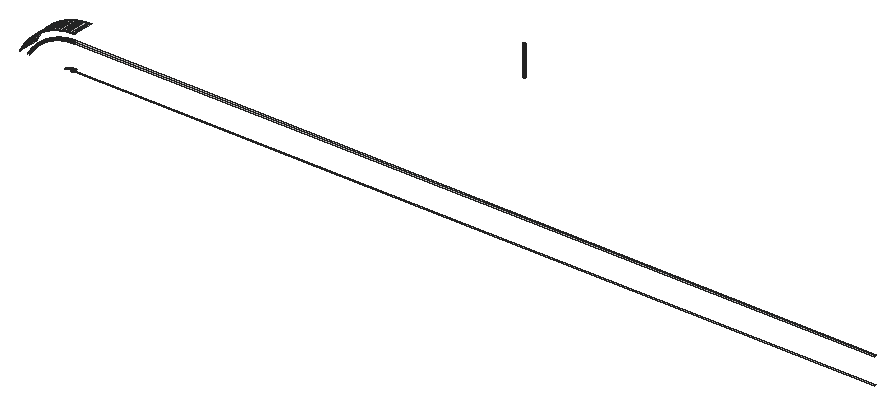
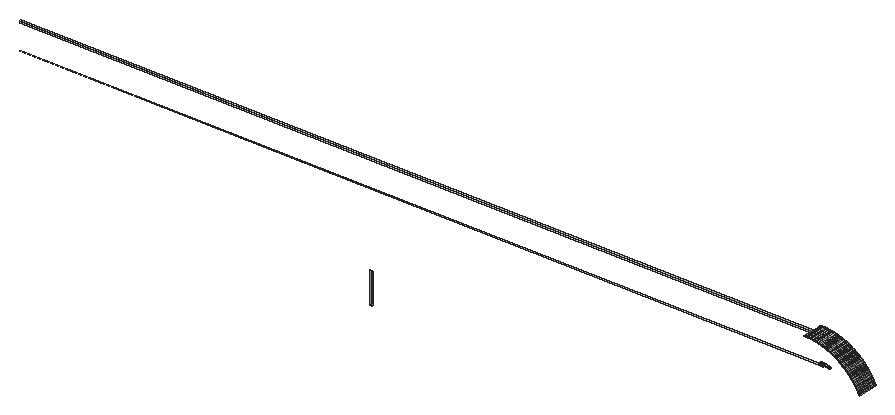
# SketchUp Ruby script. Lengths in inches.
U = 1.inch
M = Sketchup.active_model
def pt(a) = Geom::Point3d.new(a.map { |v| v * U })
def face(e, loops, mat)
  f = e.add_face(loops[0].map { |a| pt(a) })
  loops[1..].each { |l| e.add_face(l.map { |a| pt(a) }).erase! }
  f.material = f.back_material = mat if mat
  f
end
# faces: each face lists its corners as indices into pts; further lists are holes
def faces(e, pts, list, mat = nil) = list.each { |f| face(e, (f[0].is_a?(Array) ? f : [f]).map { |l| l.map { |i| pts[i] } }, mat) }
# xy, xz, yz: faces in a plane at the given z, y or x. An outline is a flat list of corners, or four numbers for a rectangle; further outlines are holes
def ring(l) = l.size == 4 ? [[l[0], l[1]], [l[2], l[1]], [l[2], l[3]], [l[0], l[3]]] : l.each_slice(2).to_a
def flat(e, list, mat, &to3) = list.each { |f| face(e, (f[0].is_a?(Array) ? f : [f]).map { |l| ring(l).map { |u, v| to3.(u, v) } }, mat) }
def xy(e, z, list, mat = nil) = flat(e, list, mat) { |x, y| [x, y, z] }
def xz(e, y, list, mat = nil) = flat(e, list, mat) { |x, z| [x, y, z] }
def yz(e, x, list, mat = nil) = flat(e, list, mat) { |y, z| [x, y, z] }
def lines(e, pts, list) = list.each { |a, b| e.add_line(pt(pts[a]), pt(pts[b])) }
# prism: a flat outline (further loops are holes) pulled along v
def prism(e, loops, v, mat = nil)
  f = face(e, loops, mat); d = Geom::Vector3d.new(v.map { |x| x * U })
  f.pushpull(f.normal.samedirection?(d) ? d.length : -d.length)
end
def box(e, o, s, mat = nil) = prism(e, [[o, [o[0] + s[0], o[1], o[2]], [o[0] + s[0], o[1] + s[1], o[2]], [o[0], o[1] + s[1], o[2]]]], [0, 0, s[2]], mat)
def at(x, y, z, deg = 0) = Geom::Transformation.translation(pt([x, y, z])) * Geom::Transformation.rotation(ORIGIN, Z_AXIS, deg.degrees)
def axes(o, x, y, z) = Geom::Transformation.new([*x, 0, *y, 0, *z, 0, *pt(o).to_a, 1])
def part(name) = M.definitions.add(name)
# library, detail: a bought-in or finely detailed component or shape, given as its bounding box
def library(name, o, s) = part(name).tap { |d| box(d.entities, o, s) }
def detail(e, o, s) = box(e.add_group.entities, o, s)
def put(e, d, t, mat = nil) = e.add_instance(d, t).tap { |i| i.material = mat if mat }
def group(e, t, mat = nil) = e.add_group.tap { |g| g.transformation = t; g.material = mat if mat }.entities
root = M.entities
M.materials.add("[Quartz Light Brown]").color = [215, 212, 212]
xy(root,99.98,[[35.12,38,35.25,39]],"[Quartz Light Brown]")
xy(root,99.99,[[35.37,38,35.5,39]],"[Quartz Light Brown]")
xy(root,100,[[35.625,38,35.75,39],[35.75,38,35.875,39],[35.875,38,36.04,39],[36.04,38,503.96,39]],"[Quartz Light Brown]")
xy(root,100.97,[[34.93,38,35.07,39]],"[Quartz Light Brown]")
xy(root,100.99,[[35.33,38,35.47,39]],"[Quartz Light Brown]")
xy(root,101,[[35.6,38,35.73,39],[35.73,38,35.87,39],[35.87,38,36.04,39]],"[Quartz Light Brown]")
xy(root,114.98,[[34.78,38,35.03,39]],"[Quartz Light Brown]")
xy(root,115,[[35.51,38,35.76,39],[35.76,38,36.01,39],[36.01,38,503.99,39]],"[Quartz Light Brown]")
xy(root,115.98,[[34.74,38,34.99,39]],"[Quartz Light Brown]")
xy(root,116,[[35.5,38,35.75,39],[35.75,38,36.01,39],[36.01,38,503.99,39]],"[Quartz Light Brown]")
xy(root,120,[[35.43,38,35.72,50],[35.72,38,36,50]],"[Quartz Light Brown]")
xz(root,143,[[215.8,114,216,132]],"[Quartz Light Brown]")
xz(root,143.01,[[215.41,114,215.61,132]],"[Quartz Light Brown]")
p = [[3.67,38,99.84],[3.8,38,100.09],[3.8,50,100.09],[3.67,50,99.84],[9.32,39,99.78],[9.32,38,99.78],
  [9.44,38,99.99],[9.44,39,99.99],[29.74,38,99.81],[29.74,39,99.81],[29.87,39,99.85],[29.87,38,99.85],
  [33.25,39,99.76],[33.25,38,99.76],[33.375,38,99.78],[33.375,39,99.78],[33.5,38,99.8],[33.5,39,99.8],
  [33.62,38,99.82],[33.62,39,99.82],[33.75,38,99.84],[33.75,39,99.84],[33.87,38,99.86],[33.87,39,99.86],
  [8.2,38,99.85],[8.2,39,99.85],[8.33,39,100.07],[8.33,38,100.07],[29.99,39,99.9],[29.99,38,99.9],
  [30.12,39,99.95],[30.12,38,99.95],[30.24,39,99.99],[30.24,38,99.99],[33.99,38,99.875],[33.99,39,99.875],
  [34.12,38,99.89],[34.12,39,99.89],[34.24,38,99.9],[34.24,39,99.9],[34.37,38,99.92],[34.37,39,99.92],
  [34.49,38,99.93],[34.49,39,99.93],[34.62,38,99.94],[34.62,39,99.94],[34.74,38,99.95],[34.74,39,99.95],
  [9.57,38,100.2],[9.57,39,100.2],[30.37,39,100.04],[30.37,38,100.04],[30.49,39,100.08],[30.49,38,100.08],
  [34.87,38,99.96],[34.87,39,99.96],[35,38,99.97],[35,39,99.97],[35.12,38,99.98],[35.12,39,99.98],
  [35.25,39,99.98],[35.25,38,99.98],[35.37,38,99.99],[35.37,39,99.99],[35.5,39,99.99],[35.5,38,99.99],
  [35.625,38,100],[35.625,39,100],[3.92,38,100.34],[3.92,50,100.34],[8.46,39,100.29],[8.46,38,100.29],
  [30.62,39,100.125],[30.62,38,100.125],[30.75,39,100.17],[30.75,38,100.17],[9.7,38,100.4],[9.7,39,100.4],
  [30.875,39,100.21],[30.875,38,100.21],[31,39,100.25],[31,38,100.25],[31.13,39,100.29],[31.13,38,100.29],
  [4.05,38,100.6],[4.05,50,100.6],[8.59,39,100.51],[8.59,38,100.51],[31.26,39,100.32],[31.26,38,100.32],
  [31.39,39,100.36],[31.39,38,100.36],[9.83,38,100.61],[9.83,39,100.61],[31.51,39,100.4],[31.51,38,100.4],
  [31.64,39,100.43],[31.64,38,100.43],[31.77,39,100.47],[31.77,38,100.47],[8.72,39,100.72],[8.72,38,100.72],
  [31.9,39,100.5],[31.9,38,100.5],[32.03,39,100.53],[32.03,38,100.53],[32.16,39,100.5625],[32.16,38,100.5625],
  [4.18,38,100.85],[4.18,50,100.85],[9.96,38,100.82],[9.96,39,100.82],[32.29,39,100.59],[32.29,38,100.59],
  [32.42,39,100.62],[32.42,38,100.62],[32.55,39,100.65],[32.55,38,100.65],[32.68,39,100.67],[32.68,38,100.67],
  [8.85,39,100.93],[8.85,38,100.93],[32.81,39,100.7],[32.81,38,100.7],[32.95,39,100.72],[32.95,38,100.72],
  [33.08,39,100.75],[33.08,38,100.75],[33.21,39,100.77],[33.21,38,100.77],[4.32,38,101.09],[4.32,50,101.09],
  [10.09,38,101.02],[10.09,39,101.02],[33.34,39,100.79],[33.34,38,100.79],[33.47,39,100.8125],[33.47,38,100.8125],
  [33.6,39,100.83],[33.6,38,100.83],[33.74,39,100.85],[33.74,38,100.85],[33.87,39,100.87],[33.87,38,100.87],
  [8.98,39,101.15],[8.98,38,101.15],[34,39,100.88],[34,38,100.88],[34.13,39,100.9],[34.13,38,100.9],
  [34.27,39,100.91],[34.27,38,100.91],[34.4,39,100.92],[34.4,38,100.92],[34.53,39,100.9375],[34.53,38,100.9375],
  [34.67,39,100.95],[34.67,38,100.95],[34.8,39,100.96],[34.8,38,100.96],[10.22,38,101.22],[10.22,39,101.22],
  [34.93,39,100.97],[34.93,38,100.97],[35.07,38,100.97],[35.07,39,100.97],[35.2,39,100.98],[35.2,38,100.98],
  [35.33,39,100.99],[35.33,38,100.99],[35.47,38,100.99],[35.47,39,100.99],[35.6,39,101],[35.6,38,101],
  [4.45,38,101.34],[4.45,50,101.34],[9.12,39,101.36],[9.12,38,101.36],[10.36,38,101.42],[10.36,39,101.42],
  [4.59,38,101.59],[4.59,50,101.59],[9.25,39,101.57],[9.25,38,101.57],[10.5,38,101.625],[10.5,39,101.625],
  [4.73,38,101.84],[4.73,50,101.84],[9.39,39,101.78],[9.39,38,101.78],[10.64,38,101.83],[10.64,39,101.83],
  [4.87,38,102.08],[4.87,50,102.08],[9.53,39,101.99],[9.53,38,101.99],[10.78,38,102.02],[10.78,39,102.02],
  [9.68,39,102.19],[9.68,38,102.19],[10.92,38,102.22],[10.92,39,102.22],[5.01,38,102.33],[5.01,50,102.33],
  [9.82,39,102.4],[9.82,38,102.4],[11.0625,38,102.42],[11.0625,39,102.42],[5.16,38,102.57],[5.16,50,102.57],
  [9.96,39,102.61],[9.96,38,102.61],[11.21,38,102.61],[11.21,39,102.61],[5.3,38,102.81],[5.3,50,102.81],
  [10.11,39,102.81],[10.11,38,102.81],[11.36,38,102.81],[11.36,39,102.81],[5.45,38,103.05],[5.45,50,103.05],
  [10.26,39,103.01],[10.26,38,103.01],[11.51,38,103],[11.51,39,103],[10.41,39,103.21],[10.41,38,103.21],
  [11.66,38,103.19],[11.66,39,103.19],[5.6,38,103.29],[5.6,50,103.29],[10.5625,39,103.41],[10.5625,38,103.41],
  [11.81,38,103.38],[11.81,39,103.38],[5.76,38,103.53],[5.76,50,103.53],[10.72,39,103.61],[10.72,38,103.61],
  [11.96,38,103.57],[11.96,39,103.57],[5.91,38,103.76],[5.91,50,103.76],[10.87,39,103.8125],[10.87,38,103.8125],
  [12.11,38,103.76],[12.11,39,103.76],[6.07,38,104],[6.07,50,104],[11.03,39,104.01],[11.03,38,104.01],
  [12.27,38,103.95],[12.27,39,103.95],[12.43,38,104.13],[12.43,39,104.13],[6.23,38,104.24],[6.23,50,104.24],
  [11.18,39,104.2],[11.18,38,104.2],[12.59,38,104.32],[12.59,39,104.32],[6.38,38,104.47],[6.38,50,104.47],
  [11.34,39,104.4],[11.34,38,104.4],[12.75,38,104.5],[12.75,39,104.5],[11.5,39,104.59],[11.5,38,104.59],
  [6.55,38,104.7],[6.55,50,104.7],[12.91,38,104.68],[12.91,39,104.68],[11.67,39,104.78],[11.67,38,104.78],
  [6.71,38,104.93],[6.71,50,104.93],[13.07,38,104.86],[13.07,39,104.86],[11.83,39,104.97],[11.83,38,104.97],
  [6.875,38,105.16],[6.875,50,105.16],[13.24,38,105.04],[13.24,39,105.04],[12,39,105.16],[12,38,105.16],
  [13.4,38,105.22],[13.4,39,105.22],[7.04,38,105.39],[7.04,50,105.39],[12.16,39,105.35],[12.16,38,105.35],
  [13.57,38,105.4],[13.57,39,105.4],[12.33,39,105.54],[12.33,38,105.54],[7.21,38,105.62],[7.21,50,105.62],
  [13.74,38,105.57],[13.74,39,105.57],[12.5,39,105.72],[12.5,38,105.72],[7.38,38,105.84],[7.38,50,105.84],
  [13.91,38,105.75],[13.91,39,105.75],[12.67,39,105.91],[12.67,38,105.91],[14.08,38,105.92],[14.08,39,105.92],
  [7.55,38,106.06],[7.55,50,106.06],[12.85,39,106.09],[12.85,38,106.09],[14.25,38,106.09],[14.25,39,106.09],
  [7.73,38,106.29],[7.73,50,106.29],[13.02,39,106.27],[13.02,38,106.27],[14.43,38,106.26],[14.43,39,106.26],
  [7.9,38,106.51],[7.9,50,106.51],[13.2,39,106.45],[13.2,38,106.45],[14.6,38,106.43],[14.6,39,106.43],
  [13.37,39,106.63],[13.37,38,106.63],[14.78,38,106.6],[14.78,39,106.6],[8.08,38,106.73],[8.08,50,106.73],
  [13.55,39,106.8],[13.55,38,106.8],[14.96,38,106.76],[14.96,39,106.76],[8.26,38,106.95],[8.26,50,106.95],
  [13.73,39,106.98],[13.73,38,106.98],[15.14,38,106.93],[15.14,39,106.93],[8.44,38,107.16],[8.44,50,107.16],
  [15.32,38,107.09],[15.32,39,107.09],[13.91,39,107.15],[13.91,38,107.15],[15.5,38,107.25],[15.5,39,107.25],
  [8.625,38,107.38],[8.625,50,107.38],[14.09,39,107.33],[14.09,38,107.33],[14.28,39,107.5],[14.28,38,107.5],
  [15.68,38,107.41],[15.68,39,107.41],[8.81,38,107.59],[8.81,50,107.59],[15.87,38,107.57],[15.87,39,107.57],
  [14.46,39,107.67],[14.46,38,107.67],[9,38,107.81],[9,50,107.81],[16.05,38,107.73],[16.05,39,107.73],
  [14.65,39,107.84],[14.65,38,107.84],[16.24,38,107.89],[16.24,39,107.89],[9.18,38,108.02],[9.18,50,108.02],
  [14.84,39,108],[14.84,38,108],[16.43,38,108.04],[16.43,39,108.04],[9.375,38,108.23],[9.375,50,108.23],
  [15.03,39,108.17],[15.03,38,108.17],[16.62,38,108.19],[16.62,39,108.19],[9.5625,38,108.4375],[9.5625,50,108.4375],
  [15.22,39,108.33],[15.22,38,108.33],[16.81,38,108.34],[16.81,39,108.34],[15.41,39,108.5],[15.41,38,108.5],
  [17,38,108.49],[17,39,108.49],[9.76,38,108.64],[9.76,50,108.64],[15.6,39,108.66],[15.6,38,108.66],
  [17.19,38,108.64],[17.19,39,108.64],[9.95,38,108.85],[9.95,50,108.85],[17.39,38,108.79],[17.39,39,108.79],
  [15.8,39,108.82],[15.8,38,108.82],[10.15,38,109.05],[10.15,50,109.05],[15.99,39,108.97],[15.99,38,108.97],
  [17.58,38,108.9375],[17.58,39,108.9375],[17.78,38,109.08],[17.78,39,109.08],[16.1875,39,109.13],[16.1875,38,109.13],
  [10.35,38,109.26],[10.35,50,109.26],[16.39,39,109.28],[16.39,38,109.28],[17.98,38,109.22],[17.98,39,109.22],
  [18.17,38,109.36],[18.17,39,109.36],[10.54,38,109.46],[10.54,50,109.46],[16.59,39,109.4375],[16.59,38,109.4375],
  [16.79,39,109.59],[16.79,38,109.59],[18.375,38,109.5],[18.375,39,109.5],[10.74,38,109.65],[10.74,50,109.65],
  [18.58,38,109.64],[18.58,39,109.64],[16.99,39,109.74],[16.99,38,109.74],[18.78,38,109.78],[18.78,39,109.78],
  [10.95,38,109.85],[10.95,50,109.85],[17.19,39,109.89],[17.19,38,109.89],[18.98,38,109.91],[18.98,39,109.91],
  [11.15,38,110.05],[11.15,50,110.05],[17.39,39,110.04],[17.39,38,110.04],[19.18,38,110.04],[19.18,39,110.04],
  [11.36,38,110.24],[11.36,50,110.24],[17.6,39,110.18],[17.6,38,110.18],[19.39,38,110.17],[19.39,39,110.17],
  [11.5625,38,110.4375],[11.5625,50,110.4375],[17.81,39,110.32],[17.81,38,110.32],[19.6,38,110.3],[19.6,39,110.3],
  [18.01,39,110.47],[18.01,38,110.47],[19.8,38,110.43],[19.8,39,110.43],[11.77,38,110.625],[11.77,50,110.625],
  [20.01,38,110.56],[20.01,39,110.56],[18.22,39,110.61],[18.22,38,110.61],[11.98,38,110.82],[11.98,50,110.82],
  [18.43,39,110.75],[18.43,38,110.75],[20.22,38,110.68],[20.22,39,110.68],[18.64,39,110.88],[18.64,38,110.88],
  [20.43,38,110.81],[20.43,39,110.81],[12.19,38,111],[12.19,50,111],[20.64,38,110.93],[20.64,39,110.93],
  [18.85,39,111.02],[18.85,38,111.02],[20.85,38,111.05],[20.85,39,111.05],[12.41,38,111.19],[12.41,50,111.19],
  [19.07,39,111.15],[19.07,38,111.15],[21.07,38,111.17],[21.07,39,111.17],[12.62,38,111.375],[12.62,50,111.375],
  [19.28,39,111.28],[19.28,38,111.28],[21.28,38,111.28],[21.28,39,111.28],[19.49,39,111.41],[19.49,38,111.41],
  [21.49,38,111.4],[21.49,39,111.4],[12.84,38,111.56],[12.84,50,111.56],[19.71,39,111.54],[19.71,38,111.54],
  [21.71,38,111.51],[21.71,39,111.51],[19.93,39,111.67],[19.93,38,111.67],[21.93,38,111.62],[21.93,39,111.62],
  [13.05,38,111.74],[13.05,50,111.74],[22.14,38,111.73],[22.14,39,111.73],[13.27,38,111.92],[13.27,50,111.92],
  [20.15,39,111.8],[20.15,38,111.8],[22.36,38,111.84],[22.36,39,111.84],[20.36,39,111.92],[20.36,38,111.92],
  [22.58,38,111.95],[22.58,39,111.95],[13.49,38,112.1],[13.49,50,112.1],[20.58,39,112.04],[20.58,38,112.04],
  [22.8,38,112.05],[22.8,39,112.05],[20.8,39,112.16],[20.8,38,112.16],[23.02,38,112.15],[23.02,39,112.15],
  [13.71,38,112.27],[13.71,50,112.27],[21.03,39,112.28],[21.03,38,112.28],[23.24,38,112.25],[23.24,39,112.25],
  [13.94,38,112.45],[13.94,50,112.45],[21.25,39,112.4],[21.25,38,112.4],[23.47,38,112.35],[23.47,39,112.35],
  [14.16,38,112.62],[14.16,50,112.62],[21.47,39,112.51],[21.47,38,112.51],[23.6875,38,112.45],[23.6875,39,112.45],
  [21.7,39,112.625],[21.7,38,112.625],[23.91,38,112.55],[23.91,39,112.55],[24.14,38,112.64],[24.14,39,112.64],
  [14.38,38,112.79],[14.38,50,112.79],[21.92,39,112.74],[21.92,38,112.74],[24.36,38,112.73],[24.36,39,112.73],
  [22.15,39,112.85],[22.15,38,112.85],[24.59,38,112.82],[24.59,39,112.82],[14.61,38,112.96],[14.61,50,112.96],
  [22.375,39,112.95],[22.375,38,112.95],[24.81,38,112.91],[24.81,39,112.91],[25.04,38,113],[25.04,39,113],
  [14.84,38,113.125],[14.84,50,113.125],[22.6,39,113.0625],[22.6,38,113.0625],[25.27,38,113.08],[25.27,39,113.08],
  [15.07,38,113.29],[15.07,50,113.29],[22.83,39,113.16],[22.83,38,113.16],[25.5,38,113.17],[25.5,39,113.17],
  [23.0625,39,113.27],[23.0625,38,113.27],[25.73,38,113.25],[25.73,39,113.25],[25.96,38,113.33],[25.96,39,113.33],
  [15.3,38,113.45],[15.3,50,113.45],[23.29,39,113.37],[23.29,38,113.37],[26.1875,38,113.41],[26.1875,39,113.41],
  [23.52,39,113.47],[23.52,38,113.47],[26.42,38,113.48],[26.42,39,113.48],[15.53,38,113.62],[15.53,50,113.62],
  [23.75,39,113.5625],[23.75,38,113.5625],[26.65,38,113.56],[26.65,39,113.56],[15.76,38,113.77],[15.76,50,113.77],
  [23.99,39,113.66],[23.99,38,113.66],[26.88,38,113.63],[26.88,39,113.63],[27.12,38,113.7],[27.12,39,113.7],
  [24.22,39,113.75],[24.22,38,113.75],[27.35,38,113.77],[27.35,39,113.77],[16,38,113.93],[16,50,113.93],
  [24.45,39,113.84],[24.45,38,113.84],[24.6875,39,113.93],[24.6875,38,113.93],[27.59,38,113.84],[27.59,39,113.84],
  [27.82,38,113.9],[27.82,39,113.9],[16.24,38,114.09],[16.24,50,114.09],[24.92,39,114.02],[24.92,38,114.02],
  [28.06,38,113.96],[28.06,39,113.96],[25.16,39,114.11],[25.16,38,114.11],[28.29,38,114.03],[28.29,39,114.03],
  [28.53,38,114.09],[28.53,39,114.09],[214.63,143.0625,132],[214.63,143.0625,114],[214.82,143.05,114],[214.82,143.05,132],
  [215.02,143.03,114],[215.02,143.03,132],[215.21,143.02,114],[215.21,143.02,132],[215.41,143.01,114],[215.41,143.01,132],
  [215.61,143.01,132],[215.61,143.01,114],[215.8,143,114],[215.8,143,132],[213.85,143.16,132],[213.85,143.16,114],
  [214.04,143.13,114],[214.04,143.13,132],[214.24,143.1,114],[214.24,143.1,132],[214.43,143.08,114],[214.43,143.08,132],
  [16.47,38,114.24],[16.47,50,114.24],[25.4,39,114.19],[25.4,38,114.19],[28.76,38,114.14],[28.76,39,114.14],
  [29,38,114.2],[29,39,114.2],[16.71,38,114.4],[16.71,50,114.4],[25.63,39,114.27],[25.63,38,114.27],
  [29.24,38,114.25],[29.24,39,114.25],[25.87,39,114.36],[25.87,38,114.36],[29.48,38,114.31],[29.48,39,114.31],
  [29.71,38,114.36],[29.71,39,114.36],[16.95,38,114.55],[16.95,50,114.55],[26.11,39,114.43],[26.11,38,114.43],
  [26.35,39,114.51],[26.35,38,114.51],[29.95,38,114.4],[29.95,39,114.4],[30.19,38,114.45],[30.19,39,114.45],
  [17.19,38,114.7],[17.19,50,114.7],[26.59,39,114.59],[26.59,38,114.59],[30.43,38,114.5],[30.43,39,114.5],
  [30.67,38,114.54],[30.67,39,114.54],[30.91,38,114.58],[30.91,39,114.58],[26.83,39,114.66],[26.83,38,114.66],
  [31.15,38,114.62],[31.15,39,114.62],[31.39,38,114.66],[31.39,39,114.66],[17.43,38,114.84],[17.43,50,114.84],
  [27.07,39,114.73],[27.07,38,114.73],[27.3125,39,114.8],[27.3125,38,114.8],[31.63,38,114.69],[31.63,39,114.69],
  [31.875,38,114.72],[31.875,39,114.72],[32.11,38,114.76],[32.11,39,114.76],[17.67,38,114.99],[17.67,50,114.99],
  [27.56,39,114.87],[27.56,38,114.87],[32.36,38,114.79],[32.36,39,114.79],[32.6,38,114.8125],[32.6,39,114.8125],
  [32.84,38,114.84],[32.84,39,114.84],[33.08,38,114.86],[33.08,39,114.86],[27.8,39,114.93],[27.8,38,114.93],
  [28.04,39,114.99],[28.04,38,114.99],[33.33,38,114.88],[33.33,39,114.88],[33.57,38,114.9],[33.57,39,114.9],
  [33.8125,38,114.92],[33.8125,39,114.92],[34.05,38,114.9375],[34.05,39,114.9375],[34.3,38,114.95],[34.3,39,114.95],
  [17.92,38,115.13],[17.92,50,115.13],[28.29,39,115.06],[28.29,38,115.06],[34.54,38,114.97],[34.54,39,114.97],
  [34.78,38,114.98],[34.78,39,114.98],[35.03,39,114.98],[35.03,38,114.98],[35.27,38,114.99],[35.27,39,114.99],
  [35.51,38,115],[35.51,39,115],[18.16,38,115.27],[18.16,50,115.27],[28.53,39,115.12],[28.53,38,115.12],
  [28.77,39,115.17],[28.77,38,115.17],[29.02,39,115.23],[29.02,38,115.23],[29.26,39,115.28],[29.26,38,115.28],
  [18.41,38,115.41],[18.41,50,115.41],[29.51,39,115.34],[29.51,38,115.34],[29.76,39,115.39],[29.76,38,115.39],
  [18.66,38,115.55],[18.66,50,115.55],[30,39,115.43],[30,38,115.43],[30.25,39,115.48],[30.25,38,115.48],
  [18.91,38,115.68],[18.91,50,115.68],[30.5,39,115.52],[30.5,38,115.52],[30.75,39,115.57],[30.75,38,115.57],
  [30.99,39,115.61],[30.99,38,115.61],[31.24,39,115.64],[31.24,38,115.64],[31.49,39,115.68],[31.49,38,115.68],
  [19.15,38,115.82],[19.15,50,115.82],[31.74,39,115.72],[31.74,38,115.72],[31.99,39,115.75],[31.99,38,115.75],
  [32.24,39,115.78],[32.24,38,115.78],[19.4,38,115.95],[19.4,50,115.95],[32.49,39,115.81],[32.49,38,115.81],
  [32.74,39,115.83],[32.74,38,115.83],[32.99,39,115.86],[32.99,38,115.86],[19.66,38,116.08],[19.66,50,116.08],
  [33.24,39,115.88],[33.24,38,115.88],[33.49,39,115.9],[33.49,38,115.9],[33.74,39,115.92],[33.74,38,115.92],
  [33.99,39,115.9375],[33.99,38,115.9375],[34.24,39,115.95],[34.24,38,115.95],[34.49,39,115.96],[34.49,38,115.96],
  [34.74,39,115.98],[34.74,38,115.98],[34.99,38,115.98],[34.99,39,115.98],[35.25,39,115.99],[35.25,38,115.99],
  [35.5,39,116],[35.5,38,116],[19.91,38,116.2],[19.91,50,116.2],[20.16,38,116.33],[20.16,50,116.33],
  [20.42,38,116.45],[20.42,50,116.45],[20.67,38,116.57],[20.67,50,116.57],[20.93,38,116.69],[20.93,50,116.69],
  [21.19,38,116.8125],[21.19,50,116.8125],[21.44,38,116.93],[21.44,50,116.93],[21.7,38,117.04],[21.7,50,117.04],
  [21.96,38,117.15],[21.96,50,117.15],[22.22,38,117.26],[22.22,50,117.26],[22.49,38,117.37],[22.49,50,117.37],
  [22.75,38,117.47],[22.75,50,117.47],[23.01,38,117.58],[23.01,50,117.58],[23.27,38,117.68],[23.27,50,117.68],
  [23.54,38,117.77],[23.54,50,117.77],[23.81,38,117.87],[23.81,50,117.87],[24.07,38,117.97],[24.07,50,117.97],
  [24.34,38,118.06],[24.34,50,118.06],[24.61,38,118.15],[24.61,50,118.15],[24.875,38,118.24],[24.875,50,118.24],
  [25.14,38,118.32],[25.14,50,118.32],[25.41,38,118.41],[25.41,50,118.41],[25.69,38,118.49],[25.69,50,118.49],
  [25.96,38,118.57],[25.96,50,118.57],[26.23,38,118.65],[26.23,50,118.65],[26.5,38,118.72],[26.5,50,118.72],
  [26.77,38,118.8],[26.77,50,118.8],[27.05,38,118.87],[27.05,50,118.87],[27.32,38,118.9375],[27.32,50,118.9375],
  [27.6,38,119.01],[27.6,50,119.01],[27.87,38,119.07],[27.87,50,119.07],[28.15,38,119.13],[28.15,50,119.13],
  [28.42,38,119.19],[28.42,50,119.19],[28.7,38,119.25],[28.7,50,119.25],[28.98,38,119.31],[28.98,50,119.31],
  [29.25,38,119.36],[29.25,50,119.36],[29.53,38,119.41],[29.53,50,119.41],[29.8125,38,119.46],[29.8125,50,119.46],
  [30.09,38,119.51],[30.09,50,119.51],[30.37,38,119.56],[30.37,50,119.56],[30.65,38,119.6],[30.65,50,119.6],
  [30.93,38,119.64],[30.93,50,119.64],[31.21,38,119.68],[31.21,50,119.68],[31.49,38,119.72],[31.49,50,119.72],
  [31.77,38,119.75],[31.77,50,119.75],[32.05,38,119.78],[32.05,50,119.78],[32.33,38,119.8125],[32.33,50,119.8125],
  [32.61,38,119.84],[32.61,50,119.84],[32.89,38,119.87],[32.89,50,119.87],[33.18,38,119.89],[33.18,50,119.89],
  [33.46,38,119.91],[33.46,50,119.91],[33.74,38,119.93],[33.74,50,119.93],[34.02,38,119.95],[34.02,50,119.95],
  [34.3,38,119.96],[34.3,50,119.96],[34.59,38,119.97],[34.59,50,119.97],[34.87,38,119.98],[34.87,50,119.98],
  [35.15,38,119.99],[35.15,50,119.99],[35.43,38,120],[35.43,50,120]]
faces(root,p,[[0,1,2,3],[4,5,6,7],[8,9,10,11],[12,13,14,15],[15,14,16,17],[17,16,18,19],[19,18,20,21],[21,20,22,23],
  [24,25,26,27],[11,10,28,29],[29,28,30,31],[31,30,32,33],[23,22,34,35],[35,34,36,37],[37,36,38,39],[39,38,40,41],
  [41,40,42,43],[43,42,44,45],[45,44,46,47],[7,6,48,49],[33,32,50,51],[51,50,52,53],[47,46,54,55],[55,54,56,57],
  [57,56,58,59],[60,61,62,63],[64,65,66,67],[1,68,69,2],[27,26,70,71],[53,52,72,73],[73,72,74,75],[49,48,76,77],
  [75,74,78,79],[79,78,80,81],[81,80,82,83],[68,84,85,69],[71,70,86,87],[83,82,88,89],[89,88,90,91],[77,76,92,93],
  [91,90,94,95],[95,94,96,97],[97,96,98,99],[87,86,100,101],[99,98,102,103],[103,102,104,105],[105,104,106,107],[84,108,109,85],
  [93,92,110,111],[107,106,112,113],[113,112,114,115],[115,114,116,117],[117,116,118,119],[101,100,120,121],[119,118,122,123],[123,122,124,125],
  [125,124,126,127],[127,126,128,129],[108,130,131,109],[111,110,132,133],[129,128,134,135],[135,134,136,137],[137,136,138,139],[139,138,140,141],
  [141,140,142,143],[121,120,144,145],[143,142,146,147],[147,146,148,149],[149,148,150,151],[151,150,152,153],[153,152,154,155],[155,154,156,157],
  [157,156,158,159],[133,132,160,161],[159,158,162,163],[164,165,166,167],[167,166,168,169],[170,171,172,173],[130,174,175,131],[145,144,176,177],
  [161,160,178,179],[174,180,181,175],[177,176,182,183],[179,178,184,185],[180,186,187,181],[183,182,188,189],[185,184,190,191],[186,192,193,187],
  [189,188,194,195],[191,190,196,197],[195,194,198,199],[197,196,200,201],[192,202,203,193],[199,198,204,205],[201,200,206,207],[202,208,209,203],
  [205,204,210,211],[207,206,212,213],[208,214,215,209],[211,210,216,217],[213,212,218,219],[214,220,221,215],[217,216,222,223],[219,218,224,225],
  [223,222,226,227],[225,224,228,229],[220,230,231,221],[227,226,232,233],[229,228,234,235],[230,236,237,231],[233,232,238,239],[235,234,240,241],
  [236,242,243,237],[239,238,244,245],[241,240,246,247],[242,248,249,243],[245,244,250,251],[247,246,252,253],[253,252,254,255],[248,256,257,249],
  [251,250,258,259],[255,254,260,261],[256,262,263,257],[259,258,264,265],[261,260,266,267],[265,264,268,269],[262,270,271,263],[267,266,272,273],
  [269,268,274,275],[270,276,277,271],[273,272,278,279],[275,274,280,281],[276,282,283,277],[279,278,284,285],[281,280,286,287],[285,284,288,289],
  [282,290,291,283],[287,286,292,293],[289,288,294,295],[293,292,296,297],[290,298,299,291],[295,294,300,301],[297,296,302,303],[298,304,305,299],
  [301,300,306,307],[303,302,308,309],[307,306,310,311],[304,312,313,305],[309,308,314,315],[311,310,316,317],[312,318,319,313],[315,314,320,321],
  [317,316,322,323],[318,324,325,319],[321,320,326,327],[323,322,328,329],[327,326,330,331],[329,328,332,333],[324,334,335,325],[331,330,336,337],
  [333,332,338,339],[334,340,341,335],[337,336,342,343],[339,338,344,345],[340,346,347,341],[345,344,348,349],[343,342,350,351],[349,348,352,353],
  [346,354,355,347],[351,350,356,357],[357,356,358,359],[353,352,360,361],[354,362,363,355],[361,360,364,365],[359,358,366,367],[362,368,369,363],
  [365,364,370,371],[367,366,372,373],[371,370,374,375],[368,376,377,369],[373,372,378,379],[375,374,380,381],[376,382,383,377],[379,378,384,385],
  [381,380,386,387],[382,388,389,383],[385,384,390,391],[387,386,392,393],[391,390,394,395],[393,392,396,397],[388,398,399,389],[395,394,400,401],
  [397,396,402,403],[398,404,405,399],[403,402,406,407],[401,400,408,409],[404,410,411,405],[409,408,412,413],[407,406,414,415],[415,414,416,417],
  [413,412,418,419],[410,420,421,411],[419,418,422,423],[417,416,424,425],[425,424,426,427],[420,428,429,421],[423,422,430,431],[431,430,432,433],
  [427,426,434,435],[428,436,437,429],[435,434,438,439],[433,432,440,441],[439,438,442,443],[436,444,445,437],[441,440,446,447],[443,442,448,449],
  [444,450,451,445],[447,446,452,453],[449,448,454,455],[450,456,457,451],[453,452,458,459],[455,454,460,461],[456,462,463,457],[459,458,464,465],
  [461,460,466,467],[465,464,468,469],[467,466,470,471],[462,472,473,463],[471,470,474,475],[469,468,476,477],[472,478,479,473],[477,476,480,481],
  [475,474,482,483],[481,480,484,485],[483,482,486,487],[478,488,489,479],[487,486,490,491],[485,484,492,493],[491,490,494,495],[488,496,497,489],
  [493,492,498,499],[495,494,500,501],[496,502,503,497],[499,498,504,505],[501,500,506,507],[505,504,508,509],[507,506,510,511],[502,512,513,503],
  [509,508,514,515],[511,510,516,517],[515,514,518,519],[517,516,520,521],[512,522,523,513],[521,520,524,525],[522,526,527,523],[519,518,528,529],
  [525,524,530,531],[529,528,532,533],[531,530,534,535],[526,536,537,527],[533,532,538,539],[535,534,540,541],[539,538,542,543],[541,540,544,545],
  [536,546,547,537],[543,542,548,549],[545,544,550,551],[546,552,553,547],[549,548,554,555],[551,550,556,557],[552,558,559,553],[555,554,560,561],
  [557,556,562,563],[561,560,564,565],[563,562,566,567],[567,566,568,569],[558,570,571,559],[565,564,572,573],[569,568,574,575],[573,572,576,577],
  [575,574,578,579],[570,580,581,571],[577,576,582,583],[579,578,584,585],[585,584,586,587],[580,588,589,581],[583,582,590,591],[587,586,592,593],
  [588,594,595,589],[591,590,596,597],[593,592,598,599],[597,596,600,601],[599,598,602,603],[603,602,604,605],[594,606,607,595],[601,600,608,609],
  [605,604,610,611],[609,608,612,613],[611,610,614,615],[606,616,617,607],[613,612,618,619],[615,614,620,621],[616,622,623,617],[619,618,624,625],
  [621,620,626,627],[627,626,628,629],[625,624,630,631],[629,628,632,633],[622,634,635,623],[631,630,636,637],[637,636,638,639],[633,632,640,641],
  [641,640,642,643],[634,644,645,635],[639,638,646,647],[643,642,648,649],[647,646,650,651],[649,648,652,653],[653,652,654,655],[656,657,658,659],
  [659,658,660,661],[661,660,662,663],[663,662,664,665],[666,667,668,669],[670,671,672,673],[673,672,674,675],[675,674,676,677],[677,676,657,656],
  [644,678,679,645],[651,650,680,681],[655,654,682,683],[683,682,684,685],[678,686,687,679],[681,680,688,689],[685,684,690,691],[689,688,692,693],
  [691,690,694,695],[695,694,696,697],[686,698,699,687],[693,692,700,701],[701,700,702,703],[697,696,704,705],[705,704,706,707],[698,708,709,699],
  [703,702,710,711],[707,706,712,713],[713,712,714,715],[715,714,716,717],[711,710,718,719],[717,716,720,721],[721,720,722,723],[708,724,725,709],
  [719,718,726,727],[727,726,728,729],[723,722,730,731],[731,730,732,733],[733,732,734,735],[724,736,737,725],[729,728,738,739],[735,734,740,741],
  [741,740,742,743],[743,742,744,745],[745,744,746,747],[739,738,748,749],[749,748,750,751],[747,746,752,753],[753,752,754,755],[755,754,756,757],
  [757,756,758,759],[759,758,760,761],[736,762,763,737],[751,750,764,765],[761,760,766,767],[767,766,768,769],[770,771,772,773],[773,772,774,775],
  [762,776,777,763],[765,764,778,779],[779,778,780,781],[781,780,782,783],[783,782,784,785],[776,786,787,777],[785,784,788,789],[789,788,790,791],
  [786,792,793,787],[791,790,794,795],[795,794,796,797],[792,798,799,793],[797,796,800,801],[801,800,802,803],[803,802,804,805],[805,804,806,807],
  [807,806,808,809],[798,810,811,799],[809,808,812,813],[813,812,814,815],[815,814,816,817],[810,818,819,811],[817,816,820,821],[821,820,822,823],
  [823,822,824,825],[818,826,827,819],[825,824,828,829],[829,828,830,831],[831,830,832,833],[833,832,834,835],[835,834,836,837],[837,836,838,839],
  [839,838,840,841],[842,843,844,845],[845,844,846,847],[826,848,849,827],[848,850,851,849],[850,852,853,851],[852,854,855,853],[854,856,857,855],
  [856,858,859,857],[858,860,861,859],[860,862,863,861],[862,864,865,863],[864,866,867,865],[866,868,869,867],[868,870,871,869],[870,872,873,871],
  [872,874,875,873],[874,876,877,875],[876,878,879,877],[878,880,881,879],[880,882,883,881],[882,884,885,883],[884,886,887,885],[886,888,889,887],
  [888,890,891,889],[890,892,893,891],[892,894,895,893],[894,896,897,895],[896,898,899,897],[898,900,901,899],[900,902,903,901],[902,904,905,903],
  [904,906,907,905],[906,908,909,907],[908,910,911,909],[910,912,913,911],[912,914,915,913],[914,916,917,915],[916,918,919,917],[918,920,921,919],
  [920,922,923,921],[922,924,925,923],[924,926,927,925],[926,928,929,927],[928,930,931,929],[930,932,933,931],[932,934,935,933],[934,936,937,935],
  [936,938,939,937],[938,940,941,939],[940,942,943,941],[942,944,945,943],[944,946,947,945],[946,948,949,947],[948,950,951,949],[950,952,953,951],
  [952,954,955,953],[954,956,957,955],[956,958,959,957],[958,960,961,959],[960,962,963,961]],"[Quartz Light Brown]")
